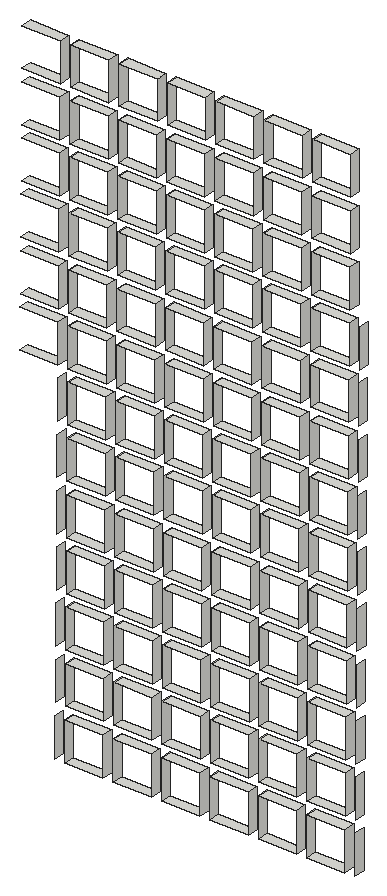
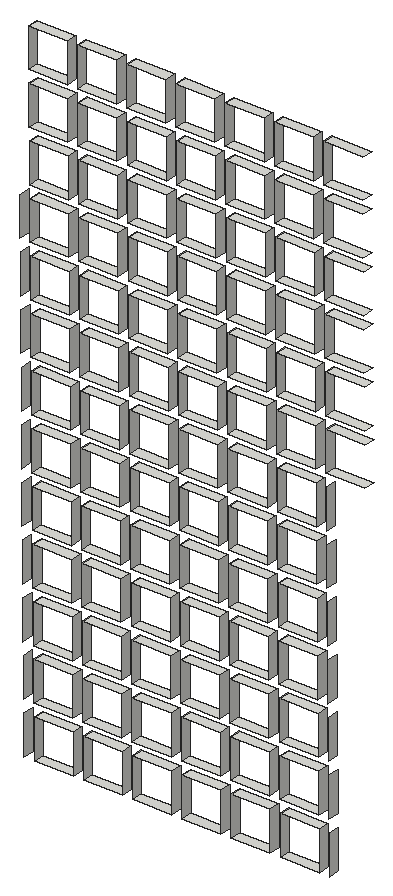
# SketchUp Ruby script. Lengths in inches.
U = 1.inch
M = Sketchup.active_model
def pt(a) = Geom::Point3d.new(a.map { |v| v * U })
def face(e, loops, mat)
  f = e.add_face(loops[0].map { |a| pt(a) })
  loops[1..].each { |l| e.add_face(l.map { |a| pt(a) }).erase! }
  f.material = f.back_material = mat if mat
  f
end
# faces: each face lists its corners as indices into pts; further lists are holes
def faces(e, pts, list, mat = nil) = list.each { |f| face(e, (f[0].is_a?(Array) ? f : [f]).map { |l| l.map { |i| pts[i] } }, mat) }
# xy, xz, yz: faces in a plane at the given z, y or x. An outline is a flat list of corners, or four numbers for a rectangle; further outlines are holes
def ring(l) = l.size == 4 ? [[l[0], l[1]], [l[2], l[1]], [l[2], l[3]], [l[0], l[3]]] : l.each_slice(2).to_a
def flat(e, list, mat, &to3) = list.each { |f| face(e, (f[0].is_a?(Array) ? f : [f]).map { |l| ring(l).map { |u, v| to3.(u, v) } }, mat) }
def xy(e, z, list, mat = nil) = flat(e, list, mat) { |x, y| [x, y, z] }
def xz(e, y, list, mat = nil) = flat(e, list, mat) { |x, z| [x, y, z] }
def yz(e, x, list, mat = nil) = flat(e, list, mat) { |y, z| [x, y, z] }
def lines(e, pts, list) = list.each { |a, b| e.add_line(pt(pts[a]), pt(pts[b])) }
# prism: a flat outline (further loops are holes) pulled along v
def prism(e, loops, v, mat = nil)
  f = face(e, loops, mat); d = Geom::Vector3d.new(v.map { |x| x * U })
  f.pushpull(f.normal.samedirection?(d) ? d.length : -d.length)
end
def box(e, o, s, mat = nil) = prism(e, [[o, [o[0] + s[0], o[1], o[2]], [o[0] + s[0], o[1] + s[1], o[2]], [o[0], o[1] + s[1], o[2]]]], [0, 0, s[2]], mat)
def at(x, y, z, deg = 0) = Geom::Transformation.translation(pt([x, y, z])) * Geom::Transformation.rotation(ORIGIN, Z_AXIS, deg.degrees)
def axes(o, x, y, z) = Geom::Transformation.new([*x, 0, *y, 0, *z, 0, *pt(o).to_a, 1])
def part(name) = M.definitions.add(name)
# library, detail: a bought-in or finely detailed component or shape, given as its bounding box
def library(name, o, s) = part(name).tap { |d| box(d.entities, o, s) }
def detail(e, o, s) = box(e.add_group.entities, o, s)
def put(e, d, t, mat = nil) = e.add_instance(d, t).tap { |i| i.material = mat if mat }
def group(e, t, mat = nil) = e.add_group.tap { |g| g.transformation = t; g.material = mat if mat }.entities
root = M.entities
xy(root,265.77,[[470.65,480.14,472.96,480.77],[473.56,480.14,475.87,480.77],[476.47,480.14,478.79,480.77],[479.38,480.14,481.7,480.77],[482.3,480.14,484.61,480.77],
  [485.21,480.14,487.52,480.77]])
xy(root,268.09,[[470.65,480.14,472.96,480.77],[473.56,480.14,475.87,480.77],[476.47,480.14,478.79,480.77],[479.38,480.14,481.7,480.77],[482.3,480.14,484.61,480.77],
  [485.21,480.14,487.52,480.77]])
xy(root,268.82,[[470.68,480.14,472.99,480.77],[473.59,480.14,475.9,480.77],[476.5,480.14,478.8125,480.77],[479.41,480.14,481.73,480.77],[482.33,480.14,484.64,480.77],
  [485.24,480.14,487.55,480.77]])
xy(root,271.13,[[470.68,480.14,472.99,480.77],[473.59,480.14,475.9,480.77],[476.5,480.14,478.8125,480.77],[479.41,480.14,481.73,480.77],[482.33,480.14,484.64,480.77],
  [485.24,480.14,487.55,480.77]])
xy(root,271.86,[[470.71,480.14,473.02,480.77],[473.62,480.14,475.93,480.77],[476.53,480.14,478.84,480.77],[479.44,480.14,481.76,480.77],[482.35,480.14,484.67,480.77],
  [485.27,480.14,487.58,480.77]])
xy(root,274.17,[[470.71,480.14,473.02,480.77],[473.62,480.14,475.93,480.77],[476.53,480.14,478.84,480.77],[479.44,480.14,481.76,480.77],[482.35,480.14,484.67,480.77],
  [485.27,480.14,487.58,480.77]])
xy(root,274.91,[[470.74,480.14,473.05,480.77],[473.65,480.14,475.96,480.77],[476.56,480.14,478.87,480.77],[479.47,480.14,481.78,480.77],[482.38,480.14,484.7,480.77],
  [485.3,480.14,487.61,480.77]])
xy(root,277.22,[[470.74,480.14,473.05,480.77],[473.65,480.14,475.96,480.77],[476.56,480.14,478.87,480.77],[479.47,480.14,481.78,480.77],[482.38,480.14,484.7,480.77],
  [485.3,480.14,487.61,480.77]])
xy(root,277.95,[[470.76,480.14,473.08,480.77],[473.68,480.14,475.99,480.77],[476.59,480.14,478.9,480.77],[479.5,480.14,481.8125,480.77],[482.41,480.14,484.73,480.77],
  [485.32,480.14,487.64,480.77]])
xy(root,280.26,[[470.76,480.14,473.08,480.77],[473.68,480.14,475.99,480.77],[476.59,480.14,478.9,480.77],[479.5,480.14,481.8125,480.77],[482.41,480.14,484.73,480.77],
  [485.32,480.14,487.64,480.77]])
xy(root,281,[[470.79,480.14,473.11,480.77],[473.71,480.14,476.02,480.77],[476.62,480.14,478.93,480.77],[479.53,480.14,481.84,480.77],[482.44,480.14,484.75,480.77],
  [485.35,480.14,487.67,480.77]])
xy(root,283.31,[[470.79,480.14,473.11,480.77],[473.71,480.14,476.02,480.77],[476.62,480.14,478.93,480.77],[479.53,480.14,481.84,480.77],[482.44,480.14,484.75,480.77],
  [485.35,480.14,487.67,480.77]])
xy(root,284.04,[[470.82,480.14,473.13,480.77],[473.73,480.14,476.05,480.77],[476.65,480.14,478.96,480.77],[479.56,480.14,481.87,480.77],[482.47,480.14,484.78,480.77],
  [485.38,480.14,487.7,480.77]])
xy(root,286.35,[[470.82,480.14,473.13,480.77],[473.73,480.14,476.05,480.77],[476.65,480.14,478.96,480.77],[479.56,480.14,481.87,480.77],[482.47,480.14,484.78,480.77],
  [485.38,480.14,487.7,480.77]])
xy(root,287.09,[[467.9375,480.14,470.25,480.77],[470.85,480.14,473.16,480.77],[473.76,480.14,476.08,480.77],[476.68,480.14,478.99,480.77],[479.59,480.14,481.9,480.77],
  [482.5,480.14,484.8125,480.77],[485.41,480.14,487.72,480.77]])
xy(root,289.4,[[467.9375,480.14,470.25,480.77],[470.85,480.14,473.16,480.77],[473.76,480.14,476.08,480.77],[476.68,480.14,478.99,480.77],[479.59,480.14,481.9,480.77],
  [482.5,480.14,484.8125,480.77],[485.41,480.14,487.72,480.77]])
xy(root,290.13,[[467.97,480.14,470.28,480.77],[470.88,480.14,473.19,480.77],[473.79,480.14,476.1,480.77],[476.7,480.14,479.02,480.77],[479.62,480.14,481.93,480.77],
  [482.53,480.14,484.84,480.77],[485.44,480.14,487.75,480.77]])
xy(root,292.44,[[467.97,480.14,470.28,480.77],[470.88,480.14,473.19,480.77],[473.79,480.14,476.1,480.77],[476.7,480.14,479.02,480.77],[479.62,480.14,481.93,480.77],
  [482.53,480.14,484.84,480.77],[485.44,480.14,487.75,480.77]])
xy(root,293.18,[[468,480.14,470.31,480.77],[470.91,480.14,473.22,480.77],[473.82,480.14,476.13,480.77],[476.73,480.14,479.05,480.77],[479.65,480.14,481.96,480.77],
  [482.56,480.14,484.87,480.77],[485.47,480.14,487.78,480.77]])
xy(root,295.49,[[468,480.14,470.31,480.77],[470.91,480.14,473.22,480.77],[473.82,480.14,476.13,480.77],[476.73,480.14,479.05,480.77],[479.65,480.14,481.96,480.77],
  [482.56,480.14,484.87,480.77],[485.47,480.14,487.78,480.77]])
xy(root,296.22,[[468.03,480.14,470.34,480.77],[470.9375,480.14,473.25,480.77],[473.85,480.14,476.16,480.77],[476.76,480.14,479.07,480.77],[479.67,480.14,481.99,480.77],
  [482.59,480.14,484.9,480.77],[485.5,480.14,487.8125,480.77]])
xy(root,298.53,[[468.03,480.14,470.34,480.77],[470.9375,480.14,473.25,480.77],[473.85,480.14,476.16,480.77],[476.76,480.14,479.07,480.77],[479.67,480.14,481.99,480.77],
  [482.59,480.14,484.9,480.77],[485.5,480.14,487.8125,480.77]])
xy(root,299.27,[[468.06,480.14,470.37,480.77],[470.97,480.14,473.28,480.77],[473.88,480.14,476.19,480.77],[476.79,480.14,479.1,480.77],[479.7,480.14,482.02,480.77],
  [482.62,480.14,484.93,480.77],[485.53,480.14,487.84,480.77]])
xy(root,301.58,[[468.06,480.14,470.37,480.77],[470.97,480.14,473.28,480.77],[473.88,480.14,476.19,480.77],[476.79,480.14,479.1,480.77],[479.7,480.14,482.02,480.77],
  [482.62,480.14,484.93,480.77],[485.53,480.14,487.84,480.77]])
xy(root,302.31,[[468.08,480.14,470.4,480.77],[471,480.14,473.31,480.77],[473.91,480.14,476.22,480.77],[476.82,480.14,479.13,480.77],[479.73,480.14,482.04,480.77],
  [482.64,480.14,484.96,480.77],[485.56,480.14,487.87,480.77]])
xy(root,304.62,[[468.08,480.14,470.4,480.77],[471,480.14,473.31,480.77],[473.91,480.14,476.22,480.77],[476.82,480.14,479.13,480.77],[479.73,480.14,482.04,480.77],
  [482.64,480.14,484.96,480.77],[485.56,480.14,487.87,480.77]])
yz(root,470.05,[[480.14,265.77,480.77,268.09]])
yz(root,470.08,[[480.14,268.82,480.77,271.13]])
yz(root,470.11,[[480.14,271.86,480.77,274.17]])
yz(root,470.14,[[480.14,274.91,480.77,277.22]])
yz(root,470.16,[[480.14,277.95,480.77,280.26]])
yz(root,470.19,[[480.14,281,480.77,283.31]])
yz(root,470.22,[[480.14,284.04,480.77,286.35]])
yz(root,470.25,[[480.14,287.09,480.77,289.4]])
yz(root,470.28,[[480.14,290.13,480.77,292.44]])
yz(root,470.31,[[480.14,293.18,480.77,295.49]])
yz(root,470.34,[[480.14,296.22,480.77,298.53]])
yz(root,470.37,[[480.14,299.27,480.77,301.58]])
yz(root,470.4,[[480.14,302.31,480.77,304.62]])
yz(root,470.65,[[480.14,265.77,480.77,268.09]])
yz(root,470.68,[[480.14,268.82,480.77,271.13]])
yz(root,470.71,[[480.14,271.86,480.77,274.17]])
yz(root,470.74,[[480.14,274.91,480.77,277.22]])
yz(root,470.76,[[480.14,277.95,480.77,280.26]])
yz(root,470.79,[[480.14,281,480.77,283.31]])
yz(root,470.82,[[480.14,284.04,480.77,286.35]])
yz(root,470.85,[[480.14,287.09,480.77,289.4]])
yz(root,470.88,[[480.14,290.13,480.77,292.44]])
yz(root,470.91,[[480.14,293.18,480.77,295.49]])
yz(root,470.9375,[[480.14,296.22,480.77,298.53]])
yz(root,470.97,[[480.14,299.27,480.77,301.58]])
yz(root,471,[[480.14,302.31,480.77,304.62]])
yz(root,472.96,[[480.14,265.77,480.77,268.09]])
yz(root,472.99,[[480.14,268.82,480.77,271.13]])
yz(root,473.02,[[480.14,271.86,480.77,274.17]])
yz(root,473.05,[[480.14,274.91,480.77,277.22]])
yz(root,473.08,[[480.14,277.95,480.77,280.26]])
yz(root,473.11,[[480.14,281,480.77,283.31]])
yz(root,473.13,[[480.14,284.04,480.77,286.35]])
yz(root,473.16,[[480.14,287.09,480.77,289.4]])
yz(root,473.19,[[480.14,290.13,480.77,292.44]])
yz(root,473.22,[[480.14,293.18,480.77,295.49]])
yz(root,473.25,[[480.14,296.22,480.77,298.53]])
yz(root,473.28,[[480.14,299.27,480.77,301.58]])
yz(root,473.31,[[480.14,302.31,480.77,304.62]])
yz(root,473.56,[[480.14,265.77,480.77,268.09]])
yz(root,473.59,[[480.14,268.82,480.77,271.13]])
yz(root,473.62,[[480.14,271.86,480.77,274.17]])
yz(root,473.65,[[480.14,274.91,480.77,277.22]])
yz(root,473.68,[[480.14,277.95,480.77,280.26]])
yz(root,473.71,[[480.14,281,480.77,283.31]])
yz(root,473.73,[[480.14,284.04,480.77,286.35]])
yz(root,473.76,[[480.14,287.09,480.77,289.4]])
yz(root,473.79,[[480.14,290.13,480.77,292.44]])
yz(root,473.82,[[480.14,293.18,480.77,295.49]])
yz(root,473.85,[[480.14,296.22,480.77,298.53]])
yz(root,473.88,[[480.14,299.27,480.77,301.58]])
yz(root,473.91,[[480.14,302.31,480.77,304.62]])
yz(root,475.87,[[480.14,265.77,480.77,268.09]])
yz(root,475.9,[[480.14,268.82,480.77,271.13]])
yz(root,475.93,[[480.14,271.86,480.77,274.17]])
yz(root,475.96,[[480.14,274.91,480.77,277.22]])
yz(root,475.99,[[480.14,277.95,480.77,280.26]])
yz(root,476.02,[[480.14,281,480.77,283.31]])
yz(root,476.05,[[480.14,284.04,480.77,286.35]])
yz(root,476.08,[[480.14,287.09,480.77,289.4]])
yz(root,476.1,[[480.14,290.13,480.77,292.44]])
yz(root,476.13,[[480.14,293.18,480.77,295.49]])
yz(root,476.16,[[480.14,296.22,480.77,298.53]])
yz(root,476.19,[[480.14,299.27,480.77,301.58]])
yz(root,476.22,[[480.14,302.31,480.77,304.62]])
yz(root,476.47,[[480.14,265.77,480.77,268.09]])
yz(root,476.5,[[480.14,268.82,480.77,271.13]])
yz(root,476.53,[[480.14,271.86,480.77,274.17]])
yz(root,476.56,[[480.14,274.91,480.77,277.22]])
yz(root,476.59,[[480.14,277.95,480.77,280.26]])
yz(root,476.62,[[480.14,281,480.77,283.31]])
yz(root,476.65,[[480.14,284.04,480.77,286.35]])
yz(root,476.68,[[480.14,287.09,480.77,289.4]])
yz(root,476.7,[[480.14,290.13,480.77,292.44]])
yz(root,476.73,[[480.14,293.18,480.77,295.49]])
yz(root,476.76,[[480.14,296.22,480.77,298.53]])
yz(root,476.79,[[480.14,299.27,480.77,301.58]])
yz(root,476.82,[[480.14,302.31,480.77,304.62]])
yz(root,478.79,[[480.14,265.77,480.77,268.09]])
yz(root,478.8125,[[480.14,268.82,480.77,271.13]])
yz(root,478.84,[[480.14,271.86,480.77,274.17]])
yz(root,478.87,[[480.14,274.91,480.77,277.22]])
yz(root,478.9,[[480.14,277.95,480.77,280.26]])
yz(root,478.93,[[480.14,281,480.77,283.31]])
yz(root,478.96,[[480.14,284.04,480.77,286.35]])
yz(root,478.99,[[480.14,287.09,480.77,289.4]])
yz(root,479.02,[[480.14,290.13,480.77,292.44]])
yz(root,479.05,[[480.14,293.18,480.77,295.49]])
yz(root,479.07,[[480.14,296.22,480.77,298.53]])
yz(root,479.1,[[480.14,299.27,480.77,301.58]])
yz(root,479.13,[[480.14,302.31,480.77,304.62]])
yz(root,479.38,[[480.14,265.77,480.77,268.09]])
yz(root,479.41,[[480.14,268.82,480.77,271.13]])
yz(root,479.44,[[480.14,271.86,480.77,274.17]])
yz(root,479.47,[[480.14,274.91,480.77,277.22]])
yz(root,479.5,[[480.14,277.95,480.77,280.26]])
yz(root,479.53,[[480.14,281,480.77,283.31]])
yz(root,479.56,[[480.14,284.04,480.77,286.35]])
yz(root,479.59,[[480.14,287.09,480.77,289.4]])
yz(root,479.62,[[480.14,290.13,480.77,292.44]])
yz(root,479.65,[[480.14,293.18,480.77,295.49]])
yz(root,479.67,[[480.14,296.22,480.77,298.53]])
yz(root,479.7,[[480.14,299.27,480.77,301.58]])
yz(root,479.73,[[480.14,302.31,480.77,304.62]])
yz(root,481.7,[[480.14,265.77,480.77,268.09]])
yz(root,481.73,[[480.14,268.82,480.77,271.13]])
yz(root,481.76,[[480.14,271.86,480.77,274.17]])
yz(root,481.78,[[480.14,274.91,480.77,277.22]])
yz(root,481.8125,[[480.14,277.95,480.77,280.26]])
yz(root,481.84,[[480.14,281,480.77,283.31]])
yz(root,481.87,[[480.14,284.04,480.77,286.35]])
yz(root,481.9,[[480.14,287.09,480.77,289.4]])
yz(root,481.93,[[480.14,290.13,480.77,292.44]])
yz(root,481.96,[[480.14,293.18,480.77,295.49]])
yz(root,481.99,[[480.14,296.22,480.77,298.53]])
yz(root,482.02,[[480.14,299.27,480.77,301.58]])
yz(root,482.04,[[480.14,302.31,480.77,304.62]])
yz(root,482.3,[[480.14,265.77,480.77,268.09]])
yz(root,482.33,[[480.14,268.82,480.77,271.13]])
yz(root,482.35,[[480.14,271.86,480.77,274.17]])
yz(root,482.38,[[480.14,274.91,480.77,277.22]])
yz(root,482.41,[[480.14,277.95,480.77,280.26]])
yz(root,482.44,[[480.14,281,480.77,283.31]])
yz(root,482.47,[[480.14,284.04,480.77,286.35]])
yz(root,482.5,[[480.14,287.09,480.77,289.4]])
yz(root,482.53,[[480.14,290.13,480.77,292.44]])
yz(root,482.56,[[480.14,293.18,480.77,295.49]])
yz(root,482.59,[[480.14,296.22,480.77,298.53]])
yz(root,482.62,[[480.14,299.27,480.77,301.58]])
yz(root,482.64,[[480.14,302.31,480.77,304.62]])
yz(root,484.61,[[480.14,265.77,480.77,268.09]])
yz(root,484.64,[[480.14,268.82,480.77,271.13]])
yz(root,484.67,[[480.14,271.86,480.77,274.17]])
yz(root,484.7,[[480.14,274.91,480.77,277.22]])
yz(root,484.73,[[480.14,277.95,480.77,280.26]])
yz(root,484.75,[[480.14,281,480.77,283.31]])
yz(root,484.78,[[480.14,284.04,480.77,286.35]])
yz(root,484.8125,[[480.14,287.09,480.77,289.4]])
yz(root,484.84,[[480.14,290.13,480.77,292.44]])
yz(root,484.87,[[480.14,293.18,480.77,295.49]])
yz(root,484.9,[[480.14,296.22,480.77,298.53]])
yz(root,484.93,[[480.14,299.27,480.77,301.58]])
yz(root,484.96,[[480.14,302.31,480.77,304.62]])
yz(root,485.21,[[480.14,265.77,480.77,268.09]])
yz(root,485.24,[[480.14,268.82,480.77,271.13]])
yz(root,485.27,[[480.14,271.86,480.77,274.17]])
yz(root,485.3,[[480.14,274.91,480.77,277.22]])
yz(root,485.32,[[480.14,277.95,480.77,280.26]])
yz(root,485.35,[[480.14,281,480.77,283.31]])
yz(root,485.38,[[480.14,284.04,480.77,286.35]])
yz(root,485.41,[[480.14,287.09,480.77,289.4]])
yz(root,485.44,[[480.14,290.13,480.77,292.44]])
yz(root,485.47,[[480.14,293.18,480.77,295.49]])
yz(root,485.5,[[480.14,296.22,480.77,298.53]])
yz(root,485.53,[[480.14,299.27,480.77,301.58]])
yz(root,485.56,[[480.14,302.31,480.77,304.62]])
yz(root,487.52,[[480.14,265.77,480.77,268.09]])
yz(root,487.55,[[480.14,268.82,480.77,271.13]])
yz(root,487.58,[[480.14,271.86,480.77,274.17]])
yz(root,487.61,[[480.14,274.91,480.77,277.22]])
yz(root,487.64,[[480.14,277.95,480.77,280.26]])
yz(root,487.67,[[480.14,281,480.77,283.31]])
yz(root,487.7,[[480.14,284.04,480.77,286.35]])
yz(root,487.72,[[480.14,287.09,480.77,289.4]])
yz(root,487.75,[[480.14,290.13,480.77,292.44]])
yz(root,487.78,[[480.14,293.18,480.77,295.49]])
yz(root,487.8125,[[480.14,296.22,480.77,298.53]])
yz(root,487.84,[[480.14,299.27,480.77,301.58]])
yz(root,487.87,[[480.14,302.31,480.77,304.62]])
yz(root,488.12,[[480.14,265.77,480.77,268.09]])
yz(root,488.15,[[480.14,268.82,480.77,271.13]])
yz(root,488.18,[[480.14,271.86,480.77,274.17]])
yz(root,488.21,[[480.14,274.91,480.77,277.22]])
yz(root,488.24,[[480.14,277.95,480.77,280.26]])
yz(root,488.27,[[480.14,281,480.77,283.31]])
yz(root,488.29,[[480.14,284.04,480.77,286.35]])
yz(root,488.32,[[480.14,287.09,480.77,289.4]])
yz(root,488.35,[[480.14,290.13,480.77,292.44]])
yz(root,488.38,[[480.14,293.18,480.77,295.49]])
